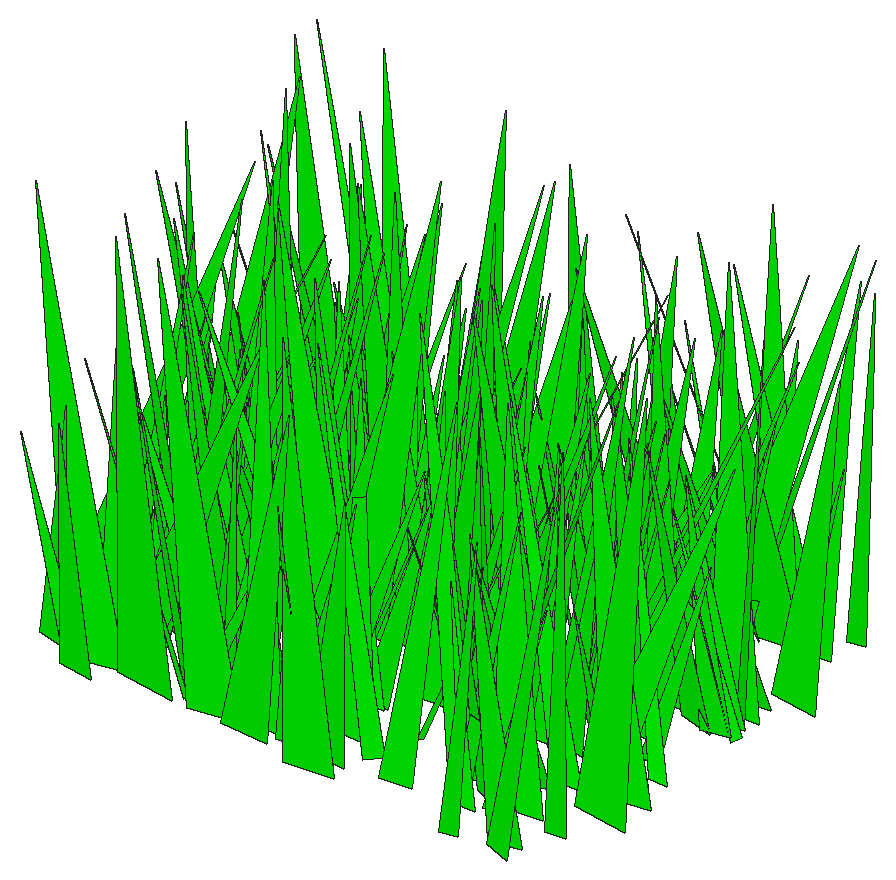
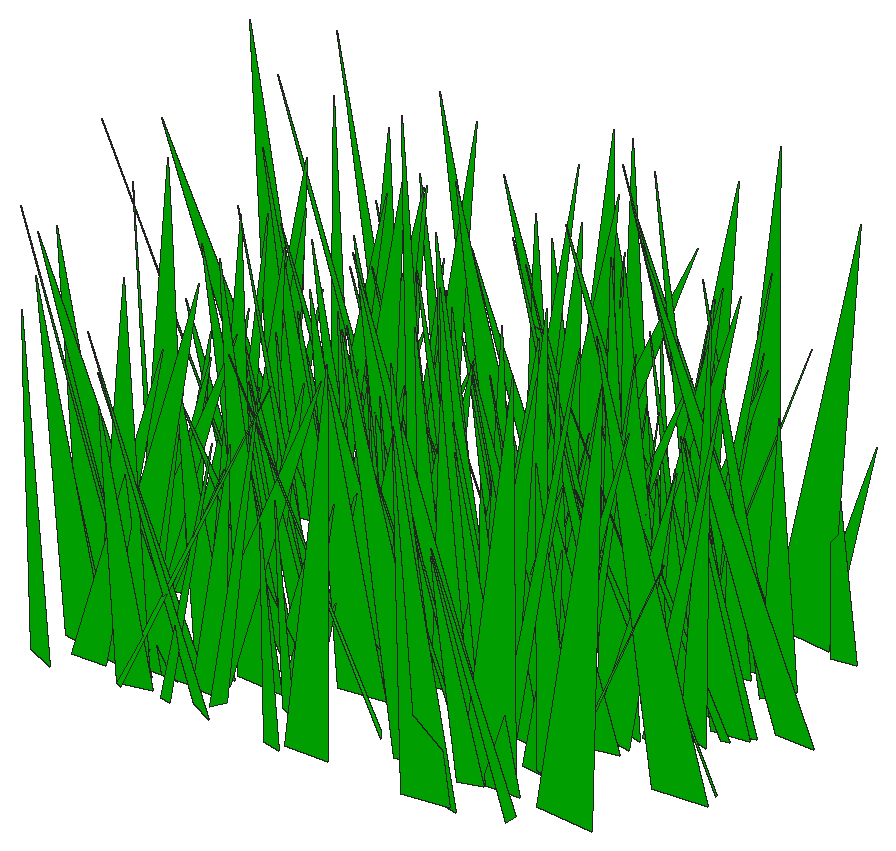
# SketchUp Ruby script. Lengths in inches.
U = 1.inch
M = Sketchup.active_model
def pt(a) = Geom::Point3d.new(a.map { |v| v * U })
def face(e, loops, mat)
  f = e.add_face(loops[0].map { |a| pt(a) })
  loops[1..].each { |l| e.add_face(l.map { |a| pt(a) }).erase! }
  f.material = f.back_material = mat if mat
  f
end
# faces: each face lists its corners as indices into pts; further lists are holes
def faces(e, pts, list, mat = nil) = list.each { |f| face(e, (f[0].is_a?(Array) ? f : [f]).map { |l| l.map { |i| pts[i] } }, mat) }
# xy, xz, yz: faces in a plane at the given z, y or x. An outline is a flat list of corners, or four numbers for a rectangle; further outlines are holes
def ring(l) = l.size == 4 ? [[l[0], l[1]], [l[2], l[1]], [l[2], l[3]], [l[0], l[3]]] : l.each_slice(2).to_a
def flat(e, list, mat, &to3) = list.each { |f| face(e, (f[0].is_a?(Array) ? f : [f]).map { |l| ring(l).map { |u, v| to3.(u, v) } }, mat) }
def xy(e, z, list, mat = nil) = flat(e, list, mat) { |x, y| [x, y, z] }
def xz(e, y, list, mat = nil) = flat(e, list, mat) { |x, z| [x, y, z] }
def yz(e, x, list, mat = nil) = flat(e, list, mat) { |y, z| [x, y, z] }
def lines(e, pts, list) = list.each { |a, b| e.add_line(pt(pts[a]), pt(pts[b])) }
# prism: a flat outline (further loops are holes) pulled along v
def prism(e, loops, v, mat = nil)
  f = face(e, loops, mat); d = Geom::Vector3d.new(v.map { |x| x * U })
  f.pushpull(f.normal.samedirection?(d) ? d.length : -d.length)
end
def box(e, o, s, mat = nil) = prism(e, [[o, [o[0] + s[0], o[1], o[2]], [o[0] + s[0], o[1] + s[1], o[2]], [o[0], o[1] + s[1], o[2]]]], [0, 0, s[2]], mat)
def at(x, y, z, deg = 0) = Geom::Transformation.translation(pt([x, y, z])) * Geom::Transformation.rotation(ORIGIN, Z_AXIS, deg.degrees)
def axes(o, x, y, z) = Geom::Transformation.new([*x, 0, *y, 0, *z, 0, *pt(o).to_a, 1])
def part(name) = M.definitions.add(name)
# library, detail: a bought-in or finely detailed component or shape, given as its bounding box
def library(name, o, s) = part(name).tap { |d| box(d.entities, o, s) }
def detail(e, o, s) = box(e.add_group.entities, o, s)
def put(e, d, t, mat = nil) = e.add_instance(d, t).tap { |i| i.material = mat if mat }
def group(e, t, mat = nil) = e.add_group.tap { |g| g.transformation = t; g.material = mat if mat }.entities
root = M.entities
M.materials.add("[0065_Lime]").color = [0, 255, 0]
c1 = part("fur_instance\#9")
p = [[0.8125,0,1.79],[0.67,-0.02,1.48],[0,-0.11,0],[0,0.11,0]]
faces(c1.entities,p,[[0,1,2,3]])
put(root,c1,axes([150.21,31.57,1.48],[1.25722,-1.1199,2.20986],[8.33837,0.21926,0.58469],[-1.17085,0.35899,6.53684]),"[0065_Lime]")
put(root,c1,axes([148.53,28.71,1.48],[1.16596,1.23629,0.95394],[-8.84406,0.14774,0.73606],[0.75159,-0.17936,7.18145]),"[0065_Lime]")
put(root,c1,axes([150.23,26.02,1.48],[6.06668,0.6304,2.794],[-4.69091,0.95672,-0.4941],[-3.14967,-0.21064,6.1175]),"[0065_Lime]")
put(root,c1,axes([151.66,29.75,1.48],[-5.19716,-0.05545,0.37346],[0.46632,-0.72225,0.69996],[0.38612,0.12586,4.18142]),"[0065_Lime]")
put(root,c1,axes([150.99,26.8,1.48],[-5.757,-0.54802,1.14363],[3.87575,-0.83147,-0.44215],[1.47149,0.04595,5.63887]),"[0065_Lime]")
put(root,c1,axes([149.74,20.19,1.48],[-1.95337,-0.61768,0.9126],[4.3473,-0.30393,-0.73637],[1.29694,0.08845,3.84276]),"[0065_Lime]")
put(root,c1,axes([150.39,22.17,1.48],[1.14069,0.81233,0.10333],[-5.7234,0.16121,-0.6625],[-0.8236,0.00482,4.74697]),"[0065_Lime]")
put(root,c1,axes([151.1,19.46,1.48],[-2.82874,0.41361,0.72305],[-3.06841,-0.39064,-0.45464],[0.1977,-0.14491,3.28939]),"[0065_Lime]")
put(root,c1,axes([149.5625,25.26,1.48],[-0.08642,0.8548,0.2891],[-6.05029,-0.01798,0.58487],[0.7252,-0.04815,4.91399]),"[0065_Lime]")
put(root,c1,axes([151.46,19.91,1.48],[-1.91109,1.18893,1.46459],[-8.63546,-0.24693,-0.73853],[-0.50999,-0.27414,7.01694]),"[0065_Lime]")
put(root,c1,axes([147.82,28.05,1.48],[6.7977,0.06806,0.24061],[-0.50567,0.95316,0.41755],[-0.2577,-0.07496,5.52761]),"[0065_Lime]")
put(root,c1,axes([149.375,25.08,1.48],[1.69963,-0.68769,1.09754],[5.06302,0.21503,-0.67286],[0.3705,0.21621,4.15998]),"[0065_Lime]")
put(root,c1,axes([148.03,24.44,1.48],[6.20339,0.92123,0.82324],[-6.63313,0.86388,0.67735],[-0.08398,-0.18379,7.3103]),"[0065_Lime]")
put(root,c1,axes([151.93,27.42,1.48],[-1.03951,-0.75241,1.22688],[5.51866,-0.11233,0.78541],[-0.70054,0.2316,4.36672]),"[0065_Lime]")
put(root,c1,axes([150.1,22.9375,1.48],[7.07255,-0.25948,1.89783],[2.19672,1.02559,-0.71773],[-2.00699,0.20815,5.90228]),"[0065_Lime]")
put(root,c1,axes([151.26,19.26,1.48],[-1.66813,-0.7076,0.17773],[4.99243,-0.2364,-0.53558],[0.69374,-0.0002,4.2816]),"[0065_Lime]")
put(root,c1,axes([152.82,29.54,1.48],[-5.91693,-0.51747,1.22347],[3.86725,-0.83703,0.51137],[0.93194,0.18795,5.64585]),"[0065_Lime]")
put(root,c1,axes([151.47,22.625,1.48],[-1.6541,0.58026,0.46138],[-4.11396,-0.24106,0.40058],[0.67048,-0.04759,3.59617]),"[0065_Lime]")
put(root,c1,axes([150.58,24.77,1.48],[0.44322,-0.57424,0.08187],[4.01648,0.05853,-0.63074],[0.76047,0.02556,3.28356]),"[0065_Lime]")
put(root,c1,axes([149.6,27.11,1.48],[3.91011,0.3967,0.2188],[-2.82089,0.53746,0.70179],[0.29127,-0.12021,3.8596]),"[0065_Lime]")
put(root,c1,axes([152.92,30.91,1.48],[-8.58835,0.29702,1.79511],[-2.03943,-1.24601,0.45255],[2.27574,0.00428,7.1801]),"[0065_Lime]")
put(root,c1,axes([149.5,25.57,1.48],[5.25428,0.28824,0.2291],[-2.06987,0.72853,0.69494],[0.05174,-0.1262,4.53512]),"[0065_Lime]")
put(root,c1,axes([152.77,27.72,1.48],[-7.60711,0.13118,1.77263],[-0.73286,-1.10889,0.66897],[2.25469,0.08217,6.19815]),"[0065_Lime]")
put(root,c1,axes([153.3,24.41,1.48],[-3.79992,-0.98927,1.54484],[7.29163,-0.51312,0.8564],[-0.05802,0.30503,6.45089]),"[0065_Lime]")
put(root,c1,axes([151.68,24.58,1.48],[-2.27555,-0.57882,0.90432],[4.13149,-0.34314,-0.48106],[1.06525,0.09437,3.79754]),"[0065_Lime]")
put(root,c1,axes([151.67,30.06,1.48],[1.69895,0.9314,0.13758],[-6.59309,0.23991,-0.55556],[-0.7036,0.00093,5.5381]),"[0065_Lime]")
put(root,c1,axes([153.14,22.14,1.48],[-7.01701,-0.40988,1.82186],[3.22627,-1.01151,0.59611],[1.76528,0.21938,6.15242]),"[0065_Lime]")
put(root,c1,axes([152.55,25.0625,1.48],[-4.44621,0.26356,0.88729],[-1.68943,-0.63982,0.76726],[1.36155,0.06678,3.84953]),"[0065_Lime]")
put(root,c1,axes([152.2,25.18,1.48],[-2.28247,0.5908,0.41408],[-4.15698,-0.32807,0.52394],[0.80995,-0.01887,3.85597]),"[0065_Lime]")
put(root,c1,axes([152.37,30.04,1.48],[1.22434,-0.58966,0.73665],[4.19745,0.19218,0.53899],[-0.90033,0.09412,3.51456]),"[0065_Lime]")
put(root,c1,axes([152.2,26.77,1.48],[5.20468,1.01749,2.17564],[-7.32825,0.79373,-0.83953],[-2.42557,-0.21476,7.20483]),"[0065_Lime]")
put(root,c1,axes([152.99,31.34,1.48],[-3.89804,1.13981,0.48533],[-8.08204,-0.55325,0.59017],[0.91298,-0.03107,7.29651]),"[0065_Lime]")
put(root,c1,axes([151.4,22.2,1.48],[2.7931,-0.51149,1.11385],[3.88515,0.37765,-0.63478],[-0.17534,0.2201,3.67771]),"[0065_Lime]")
put(root,c1,axes([151.31,32.49,1.48],[4.77893,-0.10782,0.7687],[0.96253,0.66404,-0.83809],[-0.74526,0.16622,3.8468]),"[0065_Lime]")
put(root,c1,axes([154.49,19.95,1.48],[-5.94163,-0.0114,0.58857],[0.14175,-0.83803,0.40268],[0.71419,0.07145,4.81665]),"[0065_Lime]")
put(root,c1,axes([154.0625,22.97,1.48],[-4.7246,0.83667,1.38845],[-6.15706,-0.66729,-0.38804],[0.67591,-0.23023,6.17052]),"[0065_Lime]")
put(root,c1,axes([151.69,28.04,1.48],[1.37139,0.69688,1.32194],[-5.18801,0.1564,0.79821],[0.56668,-0.25461,4.10859]),"[0065_Lime]")
put(root,c1,axes([153.34,25.2,1.48],[-5.29419,-0.13055,1.3807],[0.69726,-0.77682,-0.69241],[1.80506,-0.08284,4.317]),"[0065_Lime]")
put(root,c1,axes([153.37,22.8125,1.48],[2.15496,-0.91793,1.49343],[6.61566,0.34441,0.77743],[-1.50903,0.19908,5.54098]),"[0065_Lime]")
put(root,c1,axes([153.98,20.64,1.48],[-5.1385,-0.24778,1.28974],[2.01253,-0.73689,0.56143],[1.25422,0.16729,4.38316]),"[0065_Lime]")
put(root,c1,axes([153.22,19.78,1.48],[-2.90433,-1.24946,0.66929],[8.85228,-0.41883,-0.78424],[1.17414,0.06709,7.56824]),"[0065_Lime]")
put(root,c1,axes([154.28,29.67,1.48],[-4.98617,0.96466,0.22805],[-6.80156,-0.6999,0.81315],[0.9729,0.05094,6.85354]),"[0065_Lime]")
put(root,c1,axes([152.45,31.41,1.48],[2.76752,0.7426,1.5538],[-5.60494,0.38625,0.41954],[-0.40309,-0.2722,4.8343]),"[0065_Lime]")
put(root,c1,axes([153.29,24.38,1.48],[3.23255,1.12177,0.91797],[-7.93125,0.47314,-0.89514],[-1.44883,-0.08725,6.9483]),"[0065_Lime]")
put(root,c1,axes([155.05,20.88,1.48],[-4.22603,0.49222,0.84553],[-3.65264,-0.57489,-0.8648],[0.09461,-0.20851,4.38031]),"[0065_Lime]")
put(root,c1,axes([152.54,22.4375,1.48],[-6.65901,-0.60054,3.4818],[4.41883,-1.09385,-0.73045],[4.13056,0.20204,6.39454]),"[0065_Lime]")
put(root,c1,axes([154.57,21.95,1.48],[-4.95723,-0.58308,1.86579],[4.58455,-0.7084,0.64091],[1.20914,0.29543,5.2193]),"[0065_Lime]")
put(root,c1,axes([153.91,28.92,1.48],[1.19026,-1.17819,0.89337],[8.42049,0.17946,0.50789],[-0.77731,0.13995,6.86982]),"[0065_Lime]")
put(root,c1,axes([155,28.43,1.48],[-2.70053,0.65221,0.5112],[-4.68129,-0.37245,-0.43922],[-0.15546,-0.11436,4.34586]),"[0065_Lime]")
put(root,c1,axes([154.74,22.28,1.48],[-0.09931,0.5604,1.34787],[-4.22968,0.03441,-0.68558],[-0.87206,-0.23071,3.17172]),"[0065_Lime]")
put(root,c1,axes([153.39,31.62,1.48],[-0.93809,0.58408,0.77313],[-4.13394,-0.15809,0.68343],[1.04486,-0.10109,3.39807]),"[0065_Lime]")
put(root,c1,axes([153.47,32.93,1.48],[3.88665,0.88606,0.82098],[-6.27534,0.5607,-0.62157],[-1.18328,-0.06323,5.99301]),"[0065_Lime]")
put(root,c1,axes([153.16,28.52,1.48],[6.1171,0.38451,1.31943],[-2.62844,0.88923,-0.62084],[-1.79173,0.00826,5.41541]),"[0065_Lime]")
put(root,c1,axes([152.56,28.87,1.48],[5.63977,-0.53349,1.08494],[3.93723,0.79823,-0.38896],[-0.8316,0.16121,5.51639]),"[0065_Lime]")
put(root,c1,axes([152.04,23.66,1.48],[7.52504,-0.40401,1.05935],[3.01872,1.05939,-0.64933],[-0.92197,0.17114,6.52028]),"[0065_Lime]")
put(root,c1,axes([155.03,28.26,1.48],[0.59201,0.58476,1.08118],[-4.25043,0.12065,-0.64666],[-1.00931,-0.16507,3.3574]),"[0065_Lime]")
put(root,c1,axes([155.01,28.47,1.48],[0.96048,-1.01899,1.69173],[7.46402,0.17116,0.6507],[-1.09591,0.27264,5.91445]),"[0065_Lime]")
put(root,c1,axes([152,21.01,1.48],[4.29987,-0.9551,0.05596],[6.75404,0.59903,-0.77291],[0.76652,0.0795,6.49641]),"[0065_Lime]")
put(root,c1,axes([152.62,20.95,1.48],[8.0927,0.46333,1.06589],[-3.15987,1.14971,-0.87297],[-1.61382,0.07227,7.05431]),"[0065_Lime]")
put(root,c1,axes([153.75,33.09,1.48],[-1.62171,-1.07188,1.79012],[7.78346,-0.27686,-0.88962],[1.56469,0.26629,6.28074]),"[0065_Lime]")
put(root,c1,axes([154.79,26.18,1.48],[-4.36605,0.61742,1.11153],[-4.25765,-0.64245,0.8928],[1.74524,-0.02273,4.95874]),"[0065_Lime]")
put(root,c1,axes([155.65,19.68,1.48],[-1.94782,1.08033,2.13894],[-8.12134,-0.24672,-0.71766],[-0.25925,-0.38804,6.41123]),"[0065_Lime]")
put(root,c1,axes([153.1,25.34,1.48],[7.27364,0.40153,1.17201],[-2.80324,1.04193,-0.45087],[-1.54379,-0.00013,6.34066]),"[0065_Lime]")
put(root,c1,axes([156.43,22.8,1.48],[-3.8382,-0.58681,0.45736],[4.21143,-0.53066,0.56905],[-0.14002,0.12458,4.57844]),"[0065_Lime]")
put(root,c1,axes([154.47,21.11,1.48],[4.87225,0.34571,1.1291],[-2.24817,0.71001,-0.86587],[-1.71039,0.05154,4.3545]),"[0065_Lime]")
put(root,c1,axes([153.71,28.13,1.48],[6.11243,-0.17924,1.00481],[1.18473,0.87514,0.46261],[-1.32265,-0.04443,5.05792]),"[0065_Lime]")
put(root,c1,axes([155.28,28.05,1.48],[3.31211,0.88961,2.03434],[-6.59862,0.51558,-0.44678],[-1.67156,-0.27257,5.79464]),"[0065_Lime]")
put(root,c1,axes([155.69,22.54,1.48],[-4.01851,-0.26178,0.86011],[1.64378,-0.57937,-0.82742],[1.37355,-0.0725,3.50657]),"[0065_Lime]")
put(root,c1,axes([154.59,22.0625,1.48],[0.72977,0.78162,0.57749],[-5.58535,0.09237,0.48082],[0.49893,-0.10926,4.53795]),"[0065_Lime]")
put(root,c1,axes([155.41,20.64,1.48],[4.36716,0.41112,1.43193],[-2.78469,0.66124,-0.74241],[-1.97604,-0.02322,4.21088]),"[0065_Lime]")
put(root,c1,axes([155.51,27.97,1.48],[-1.45328,0.63254,0.23399],[-4.4581,-0.20789,0.51111],[0.68666,-0.01095,3.81356]),"[0065_Lime]")
put(root,c1,axes([156.1,26.46,1.48],[2.62887,-0.64008,1.36069],[4.52414,0.41997,0.83669],[-1.75489,0.12384,4.19535]),"[0065_Lime]")
put(root,c1,axes([153.91,24.93,1.48],[7.1511,0.42243,1.44974],[-3.22222,1.01779,0.57861],[-1.35324,-0.19119,6.2833]),"[0065_Lime]")
put(root,c1,axes([156.25,24.38,1.48],[-4.5477,-0.44224,0.78798],[3.00612,-0.6523,-0.78821],[1.34408,-0.03741,4.42899]),"[0065_Lime]")
put(root,c1,axes([156.93,24.41,1.48],[-4.25137,-0.11381,0.7346],[0.70114,-0.60795,-0.47137],[0.98995,-0.05818,3.48862]),"[0065_Lime]")
put(root,c1,axes([157.52,22.875,1.48],[-3.05967,1.15342,1.43101],[-8.39453,-0.41829,-0.57803],[-0.06673,-0.26645,7.10209]),"[0065_Lime]")
put(root,c1,axes([154.54,20.49,1.48],[4.34245,-0.25449,0.24626],[1.83456,0.60595,-0.42071],[-0.07822,0.08349,3.80391]),"[0065_Lime]")
put(root,c1,axes([155.68,27.54,1.48],[4.35013,-0.28743,1.42244],[2.42467,0.62126,-0.69959],[-1.16754,0.21925,3.84702]),"[0065_Lime]")
put(root,c1,axes([159.02,21.07,1.48],[-6.38904,0.61876,0.57947],[-4.46057,-0.88741,-0.78763],[0.03017,-0.16887,6.26235]),"[0065_Lime]")
put(root,c1,axes([154.86,30.11,1.48],[4.74666,-0.04762,0.25778],[0.273,0.65675,0.73971],[-0.37519,-0.12463,3.79949]),"[0065_Lime]")
put(root,c1,axes([157.08,27.11,1.48],[2.84865,-0.52026,1.67989],[3.77077,0.47073,0.65443],[-1.93773,0.15119,3.74309]),"[0065_Lime]")
put(root,c1,axes([155.17,31.63,1.48],[3.44929,-0.96318,1.24677],[7.02359,0.47122,-0.65808],[0.05182,0.24343,6.20689]),"[0065_Lime]")
put(root,c1,axes([157.04,23.68,1.48],[2.21239,-1.09524,0.71005],[7.7374,0.32563,0.87993],[-1.28291,0.0752,6.53144]),"[0065_Lime]")
put(root,c1,axes([155.66,25.78,1.48],[1.86242,1.23841,1.6702],[-9.03066,0.23548,0.812],[0.57982,-0.3103,7.28197]),"[0065_Lime]")
put(root,c1,axes([156.99,27.99,1.48],[-2.51417,0.7595,0.82808],[-5.38849,-0.37166,0.59783],[1.10214,-0.08453,4.81187]),"[0065_Lime]")
put(root,c1,axes([155.85,28.87,1.48],[4.03392,0.13604,0.65811],[-1.12303,0.56073,0.67048],[-0.57506,-0.14075,3.30713]),"[0065_Lime]")
put(root,c1,axes([157.08,19.9375,1.48],[-5.74935,0.79673,2.24985],[-5.78488,-0.8756,0.60916],[2.51672,-0.19253,6.53989]),"[0065_Lime]")
put(root,c1,axes([156.45,20.41,1.48],[1.33827,0.56664,0.79232],[-4.14478,0.17655,0.40096],[0.17525,-0.15141,3.43266]),"[0065_Lime]")
put(root,c1,axes([155.71,28.67,1.48],[6.76364,0.79155,0.61763],[-5.57345,0.95612,-0.67742],[-1.11578,0.02228,7.1277]),"[0065_Lime]")
put(root,c1,axes([157.82,33.09,1.48],[-2.77103,-0.97335,1.25567],[7.01497,-0.41094,-0.43147],[1.07485,0.17262,6.0532]),"[0065_Lime]")
put(root,c1,axes([157.4375,26.92,1.48],[-3.77794,-0.77552,2.00029],[5.60458,-0.60205,-0.81789],[2.25733,0.19687,5.37846]),"[0065_Lime]")
put(root,c1,axes([156.89,19.44,1.48],[1.37878,-0.99747,0.34502],[7.09084,0.18825,-0.51148],[0.53777,0.07516,5.85967]),"[0065_Lime]")
put(root,c1,axes([156.82,24.74,1.48],[4.14105,0.17888,0.24105],[-1.19709,0.5746,-0.68179],[-0.52478,0.10084,3.45737]),"[0065_Lime]")
put(root,c1,axes([157.43,27.69,1.48],[-0.93215,-0.68203,0.71127],[4.80565,-0.15372,-0.77211],[1.10852,0.09287,3.94537]),"[0065_Lime]")
put(root,c1,axes([158.05,19.77,1.48],[2.48914,0.47221,0.78327],[-3.31561,0.37154,-0.53433],[-1.10772,-0.051,3.35944]),"[0065_Lime]")
put(root,c1,axes([158,32.54,1.48],[3.85428,-0.39067,1.02302],[2.60057,0.56949,0.80481],[-1.59642,-0.01552,3.78095]),"[0065_Lime]")
put(root,c1,axes([157.66,27.73,1.48],[-3.33198,-0.73114,1.78516],[5.26432,-0.53174,-0.79654],[2.0437,0.17767,4.96225]),"[0065_Lime]")
put(root,c1,axes([157.09,26.79,1.48],[6.59633,-0.37232,1.32896],[2.57865,0.9549,0.4961],[-1.74374,0.00366,5.76091]),"[0065_Lime]")
put(root,c1,axes([159.07,29.14,1.48],[-1.36662,0.81262,1.41498],[-6.03317,-0.17268,-0.53223],[-0.26587,-0.25847,4.80419]),"[0065_Lime]")
put(root,c1,axes([158.8,22.74,1.48],[-3.81542,0.26019,0.86224],[-1.75669,-0.55629,0.48182],[1.21089,0.01279,3.41586]),"[0065_Lime]")
put(root,c1,axes([157.75,21.02,1.48],[0.08378,-0.62265,1.23264],[4.58031,-0.03347,-0.77253],[0.97556,0.21062,3.5212]),"[0065_Lime]")
put(root,c1,axes([159.17,19.1875,1.48],[-5.01131,-0.31768,1.31516],[2.15751,-0.73992,-0.54964],[1.75227,0.0025,4.43797]),"[0065_Lime]")
put(root,c1,axes([158.03,25.77,1.48],[0.62182,-1.01356,2.03113],[7.61741,0.0599,-0.54129],[0.48777,0.3566,5.864]),"[0065_Lime]")
put(root,c1,axes([157.75,29.07,1.48],[0.73601,0.92968,0.15776],[-6.56443,0.09901,0.71102],[0.84787,-0.04044,5.36795]),"[0065_Lime]")
put(root,c1,axes([157.75,29.07,1.48],[6.16283,-0.34825,1.09341],[2.3371,0.88497,0.72934],[-1.57707,-0.04944,5.35364]),"[0065_Lime]")
put(root,c1,axes([157.12,21.43,1.48],[5.37063,-0.71436,0.98527],[5.2031,0.75374,-0.45291],[-0.48931,0.17425,5.99823]),"[0065_Lime]")
put(root,c1,axes([159.49,18.94,1.48],[0.90646,1.05728,2.23153],[-7.94694,0.16683,-0.51282],[-0.99268,-0.37014,6.14313]),"[0065_Lime]")
put(root,c1,axes([159.85,31.13,1.48],[-2.02214,-0.4602,1.55049],[3.78872,-0.25099,0.77303],[0.06806,0.29914,3.03388]),"[0065_Lime]")
put(root,c1,axes([158.8125,33.35,1.48],[3.63938,-0.28882,0.70916],[1.836,0.52046,0.86867],[-1.2704,-0.07523,3.28697]),"[0065_Lime]")
put(root,c1,axes([159.07,28.38,1.48],[5.33549,-0.00441,1.71323],[-0.19852,0.80132,0.47811],[-2.09708,-0.08707,4.31362]),"[0065_Lime]")
put(root,c1,axes([159.45,21.03,1.48],[-3.7831,0.77084,1.5157],[-5.55173,-0.57174,0.57511],[1.65628,-0.15577,5.38973]),"[0065_Lime]")
put(root,c1,axes([156.92,31.03,1.48],[6.76729,0.10195,0.1585],[-0.70576,0.94782,-0.49125],[-0.25738,0.08151,5.5143]),"[0065_Lime]")
put(root,c1,axes([158.68,29.63,1.48],[0.17582,1.00315,1.97279],[-7.49282,-0.01471,0.69248],[0.83952,-0.34138,5.76727]),"[0065_Lime]")
put(root,c1,axes([160.22,29.76,1.48],[-3.48515,-0.3614,0.52969],[2.52534,-0.4982,-0.39634],[0.81321,-0.00172,3.50084]),"[0065_Lime]")
put(root,c1,axes([160.48,20.52,1.48],[-6.88774,0.31659,2.09147],[-2.67648,-1.00497,-0.73443],[2.12691,-0.2394,5.84877]),"[0065_Lime]")
put(root,c1,axes([158.57,22.91,1.48],[2.40701,-0.54403,0.87273],[4.01575,0.32054,-0.63249],[0.12021,0.18543,3.6539]),"[0065_Lime]")
put(root,c1,axes([159.36,27.35,1.48],[4.32162,0.14707,1.47428],[-1.36574,0.64092,0.50649],[-1.58591,-0.15119,3.58124]),"[0065_Lime]")
put(root,c1,axes([159.58,31.67,1.48],[3.34459,0.33392,0.8981],[-2.22283,0.49477,-0.68723],[-1.38753,0.01229,3.2658]),"[0065_Lime]")
put(root,c1,axes([159.68,23.9,1.48],[2.13037,0.80826,0.47754],[-5.70408,0.30817,-0.6417],[-0.94538,-0.03804,4.94791]),"[0065_Lime]")
put(root,c1,axes([158.33,21.3125,1.48],[4.876,-0.4389,0.67642],[3.21419,0.68071,-0.52969],[-0.34094,0.14047,4.68027]),"[0065_Lime]")
put(root,c1,axes([159.48,19.66,1.48],[-0.02954,-0.83486,0.00385],[5.90029,-0.0042,-0.56694],[0.697,0.00017,4.79943]),"[0065_Lime]")
put(root,c1,axes([160.875,23.75,1.48],[-0.21953,-0.61828,1.00526],[4.53877,-0.00911,0.46815],[-0.53595,0.17614,3.55279]),"[0065_Lime]")
put(root,c1,axes([161.34,32.46,1.48],[-6.18917,0.29467,1.32721],[-1.89256,-0.89684,0.83288],[1.86495,0.06779,5.24982]),"[0065_Lime]")
put(root,c1,axes([160.19,25.93,1.48],[-2.07009,0.78451,1.16812],[-5.58694,-0.32586,0.7825],[1.42055,-0.13838,4.77975]),"[0065_Lime]")
put(root,c1,axes([159.73,28.08,1.48],[2.82583,0.66361,1.00797],[-4.87824,0.39214,0.39764],[-0.20377,-0.18499,4.45892]),"[0065_Lime]")
put(root,c1,axes([160.02,25.77,1.48],[3.713,0.99794,0.24666],[-7.04712,0.52307,-0.72572],[-0.93084,0.0206,6.4781]),"[0065_Lime]")
put(root,c1,axes([162.45,31.36,1.48],[-3.22237,-0.82877,0.32491],[5.89725,-0.44624,0.55558],[-0.40993,0.0951,5.43851]),"[0065_Lime]")
put(root,c1,axes([160.74,24.46,1.48],[7.27768,0.70266,2.45612],[-4.97893,1.10065,-0.79013],[-3.05494,-0.11993,7.13887]),"[0065_Lime]")
put(root,c1,axes([161.88,28.5,1.48],[1.27687,-0.53222,0.84645],[3.71143,0.21382,0.80059],[-1.28595,0.08864,3.15109]),"[0065_Lime]")
put(root,c1,axes([161.99,22.64,1.48],[1.62431,0.52295,1.23034],[-3.78814,0.2757,-0.61783],[-1.33724,-0.1458,3.24467]),"[0065_Lime]")
put(root,c1,axes([164.1,33.27,1.48],[-7.10131,-0.20486,0.27162],[1.4263,-0.9961,-0.50184],[0.45012,-0.07561,5.87538]),"[0065_Lime]")
put(root,c1,axes([161.93,32.16,1.48],[1.30412,-0.636,1.13663],[4.65028,0.21067,0.41991],[-0.90197,0.16659,3.80833]),"[0065_Lime]")
put(root,c1,axes([160.4,23.77,1.48],[4.733,0.43098,1.08504],[-3.27693,0.66255,0.63916],[-0.66941,-0.19616,4.54281]),"[0065_Lime]")
put(root,c1,axes([162.48,24.92,1.48],[2.45379,-1.05185,2.01507],[7.68053,0.40131,0.83128],[-1.78315,0.2811,6.35347]),"[0065_Lime]")
put(root,c1,axes([162.6,33.14,1.48],[4.3999,-0.17063,2.14228],[0.8485,0.71877,0.7653],[-2.77324,-0.0508,3.633]),"[0065_Lime]")
put(root,c1,axes([162.84,24.55,1.48],[-0.10683,-1.0819,1.49345],[7.85264,0.0179,0.80624],[-0.99361,0.25781,6.21126]),"[0065_Lime]")
put(root,c1,axes([159.77,26.73,1.48],[7.07472,-0.30503,0.45384],[2.09949,0.99278,0.70477],[-0.7846,-0.09388,5.97807]),"[0065_Lime]")
put(root,c1,axes([163.05,21.28,1.48],[-6.45058,0.75101,1.40498],[-5.31919,-0.93551,0.59816],[1.80395,-0.07301,6.78768]),"[0065_Lime]")
put(root,c1,axes([161.14,30.95,1.48],[4.93648,-0.90033,0.47068],[6.33044,0.69806,0.81465],[-1.14583,-0.0222,6.52854]),"[0065_Lime]")
put(root,c1,axes([160.76,22.16,1.48],[4.86095,0.21201,0.17688],[-1.44213,0.67267,-0.79553],[-0.49399,0.12248,4.0629]),"[0065_Lime]")
put(root,c1,axes([163.87,21.4,1.48],[-4.27441,-0.20957,0.43597],[1.56409,-0.59276,0.59836],[0.25529,0.12276,3.63349]),"[0065_Lime]")
put(root,c1,axes([162.34,25.53,1.48],[4.70108,-0.25479,1.3267],[1.66934,0.699,0.58449],[-1.77799,-0.01739,4.0566]),"[0065_Lime]")
put(root,c1,axes([161.8,28.1875,1.48],[3.94403,-0.29272,1.22665],[2.44737,0.54639,-0.83732],[-0.78996,0.23131,3.53018]),"[0065_Lime]")
put(root,c1,axes([161.76,19.84,1.48],[6.27653,-0.56131,1.9733],[4.35736,0.90921,-0.50377],[-1.68976,0.25962,6.03067]),"[0065_Lime]")
put(root,c1,axes([163.73,25.69,1.48],[-4.32716,-0.14207,0.93109],[1.20494,-0.61452,0.56318],[0.93837,0.13398,3.57042]),"[0065_Lime]")
put(root,c1,axes([162.3,21.78,1.48],[3.99426,-0.08054,0.89401],[0.33962,0.57224,0.72347],[-1.19212,-0.10682,3.20153]),"[0065_Lime]")
put(root,c1,axes([163.44,28.15,1.48],[-0.08905,-0.71246,0.02734],[5.03606,-0.01188,0.47934],[-0.58863,0.00615,4.09688]),"[0065_Lime]")
put(root,c1,axes([162.97,22.4,1.48],[-5.24465,-0.38203,1.74047],[2.60138,-0.79542,-0.66397],[2.28097,0.02874,4.75911]),"[0065_Lime]")
put(root,c1,axes([162.41,31.25,1.48],[-0.48008,0.82158,1.03279],[-5.92595,-0.08997,0.57563],[0.82477,-0.16819,4.73702]),"[0065_Lime]")
put(root,c1,axes([164.3,32.1,1.48],[-4.3871,-0.19517,0.24351],[1.30615,-0.60772,-0.75198],[0.5592,-0.11167,3.66678]),"[0065_Lime]")
put(root,c1,axes([162.84,27.07,1.48],[3.52197,0.53755,1.0826],[-3.8503,0.52126,-0.38527],[-1.25741,-0.09048,4.21207]),"[0065_Lime]")
put(root,c1,axes([161.47,33.04,1.48],[6.36325,0.44515,0.48875],[-3.08037,0.89445,-0.7635],[-0.95299,0.08119,5.73129]),"[0065_Lime]")
put(root,c1,axes([161.53,29.14,1.48],[2.90675,0.50344,0.00324],[-3.52548,0.40179,0.67076],[0.63791,-0.07343,3.69231]),"[0065_Lime]")
put(root,c1,axes([162.43,27.37,1.48],[4.14585,0.52928,0.45365],[-3.71118,0.58759,-0.53203],[-0.85196,0.01602,4.52508]),"[0065_Lime]")
put(root,c1,axes([162.32,27.16,1.48],[6.94652,0.37767,1.39934],[-2.60208,1.00559,-0.54778],[-1.84726,0.00371,6.03376]),"[0065_Lime]")
put(root,c1,axes([164.08,20.74,1.48],[-4.04362,-0.39291,0.81055],[2.61577,-0.5835,-0.84398],[1.40328,-0.04451,3.90885]),"[0065_Lime]")
put(root,c1,axes([164.94,22.07,1.48],[-2.53062,-0.46533,0.96511],[3.51175,-0.32226,0.88587],[-0.20433,0.22448,3.27234]),"[0065_Lime]")
put(root,c1,axes([164.14,19.95,1.48],[-3.57367,0.28451,0.82857],[-1.93357,-0.52213,0.4898],[1.18252,0.00605,3.30489]),"[0065_Lime]")
put(root,c1,axes([162.79,27.81,1.48],[4.89673,0.21076,1.26247],[-1.84085,0.69011,0.8637],[-1.12682,-0.21155,4.07519]),"[0065_Lime]")
put(root,c1,axes([162.75,28.01,1.48],[4.41188,-0.1975,0.4553],[1.28236,0.61686,0.74461],[-0.8027,-0.10005,3.69205]),"[0065_Lime]")
put(root,c1,axes([165.06,32.17,1.48],[-1.98925,-1.06537,0.82494],[7.63847,-0.26885,0.5525],[-0.40606,0.16175,6.35183]),"[0065_Lime]")
put(root,c1,axes([162.36,31.875,1.48],[5.16536,0.42475,0.11361],[-2.96716,0.71858,-0.76411],[-0.59364,0.10417,4.80778]),"[0065_Lime]")
put(root,c1,axes([163.36,24.0625,1.48],[5.01452,-0.34583,1.70346],[2.85906,0.72798,-0.61626],[-1.50613,0.23052,4.50167]),"[0065_Lime]")
put(root,c1,axes([163.02,28.34,1.48],[3.76193,0.77499,1.68395],[-5.86723,0.52388,0.59332],[-0.52868,-0.29935,5.39791]),"[0065_Lime]")
put(root,c1,axes([163.69,33.08,1.48],[-1.05758,0.77565,0.51155],[-5.47512,-0.16078,0.6795],[0.94259,-0.0636,4.52089]),"[0065_Lime]")
put(root,c1,axes([165.58,32.72,1.48],[-4.80035,0.64391,1.12396],[-4.74034,-0.67761,-0.3872],[0.66117,-0.18315,5.38424]),"[0065_Lime]")
put(root,c1,axes([165.42,22.59,1.48],[-5.88284,0.57056,0.79662],[-3.95604,-0.83738,0.76785],[1.34018,0.0327,5.76342]),"[0065_Lime]")
put(root,c1,axes([163.26,32.13,1.48],[4.11136,-0.30146,0.41458],[2.0652,0.57953,0.57016],[-0.77289,-0.0551,3.72882]),"[0065_Lime]")
put(root,c1,axes([164.62,32.43,1.48],[0.91477,1.18598,0.33295],[-8.41057,0.13337,-0.63027],[-0.81515,-0.0452,6.87664]),"[0065_Lime]")
put(root,c1,axes([163.1875,25.34,1.48],[5.89541,0.66728,1.89542],[-5.09936,0.84727,0.49912],[-1.406,-0.27498,6.13735]),"[0065_Lime]")
put(root,c1,axes([163.48,20.47,1.48],[4.83151,0.46661,0.72861],[-3.20966,0.68969,-0.71819],[-1.2357,0.03295,4.71432]),"[0065_Lime]")
put(root,c1,axes([164.63,27.74,1.48],[2.57063,0.96147,1.87784],[-7.07055,0.40511,-0.54642],[-1.46795,-0.26757,5.92033]),"[0065_Lime]")
put(root,c1,axes([164.19,24.18,1.48],[-0.58799,-0.58466,1.09248],[4.2726,-0.11724,-0.58092],[0.92759,0.16941,3.36829]),"[0065_Lime]")
put(root,c1,axes([165.28,20.65,1.48],[0.01961,1.11675,0.33408],[-7.93867,0.00676,-0.44943],[-0.55427,-0.05738,6.44889]),"[0065_Lime]")
put(root,c1,axes([165.36,25.92,1.48],[1.84696,0.76569,2.19674],[-5.90868,0.31983,-0.44867],[-1.44002,-0.33026,4.65849]),"[0065_Lime]")
put(root,c1,axes([164.6,18.54,1.48],[4.33727,0.51939,1.01468],[-3.5568,0.63417,-0.81825],[-1.60246,-0.00178,4.56256]),"[0065_Lime]")
put(root,c1,axes([166.59,29.17,1.48],[-2.77663,-0.74073,0.29677],[5.27266,-0.3846,0.47298],[-0.34622,0.08329,4.82315]),"[0065_Lime]")
put(root,c1,axes([162.83,22.5,1.48],[8.23535,-0.10277,0.86549],[0.61856,1.16135,0.72687],[-1.13335,-0.11296,6.68571]),"[0065_Lime]")
put(root,c1,axes([163.23,32.11,1.48],[3.76121,1.09354,0.10024],[-7.76708,0.52612,0.50025],[0.50029,-0.05316,7.01288]),"[0065_Lime]")
put(root,c1,axes([164.58,20.29,1.48],[3.67408,0.33491,0.29663],[-2.30063,0.51489,-0.62624],[-0.72162,0.06362,3.50682]),"[0065_Lime]")
put(root,c1,axes([166.15,19.01,1.48],[1.00885,0.75296,1.36212],[-5.47515,0.18481,-0.74017],[-1.24095,-0.20325,4.37302]),"[0065_Lime]")
put(root,c1,axes([166.03,27.34,1.48],[-3.28427,-0.675,0.00443],[4.72019,-0.45365,-0.87555],[0.89159,-0.08475,4.65163]),"[0065_Lime]")
put(root,c1,axes([166.08,29.38,1.48],[3.46935,-0.23904,1.63354],[1.57387,0.56266,0.54738],[-2.10949,0.02665,3.09497]),"[0065_Lime]")
put(root,c1,axes([163.74,32.41,1.48],[8.11011,0.2031,1.09099],[-1.5884,1.14562,0.66586],[-1.16839,-0.14764,6.66766]),"[0065_Lime]")
put(root,c1,axes([166.53,23.8125,1.48],[0.93843,-0.82992,1.49377],[6.10157,0.16696,0.57221],[-1.01295,0.23686,4.83065]),"[0065_Lime]")
put(root,c1,axes([162.91,27.62,1.48],[8.60852,0.24839,0.43342],[-1.79881,1.20883,0.42507],[-0.41572,-0.0871,7.13573]),"[0065_Lime]")
put(root,c1,axes([166.97,27.77,1.48],[-3.24819,0.41663,1.03342],[-3.17568,-0.45748,-0.42401],[0.56592,-0.17582,3.55213]),"[0065_Lime]")
put(root,c1,axes([166.48,28.41,1.48],[3.88111,-0.84604,3.84178],[7.37983,0.61064,-0.42666],[-2.02398,0.60416,5.81116]),"[0065_Lime]")
put(root,c1,axes([166.75,27.28,1.48],[0.33656,-0.6227,1.35623],[4.68815,0.0767,0.41028],[-0.66263,0.22638,3.59163]),"[0065_Lime]")
put(root,c1,axes([167.25,22.85,1.48],[-1.17104,1.06089,0.41762],[-7.55222,-0.15924,-0.45654],[-0.4774,-0.08322,6.19779]),"[0065_Lime]")
put(root,c1,axes([167.41,27.36,1.48],[-4.00955,0.13486,0.80546],[-1.19075,-0.55437,-0.81172],[0.69548,-0.17168,3.25383]),"[0065_Lime]")
put(root,c1,axes([166.03,32.22,1.48],[3.31058,0.99946,0.10438],[-7.05278,0.46373,-0.78618],[-0.93011,0.04109,6.33294]),"[0065_Lime]")
put(root,c1,axes([167.21,24.24,1.48],[-5.70838,0.31833,1.36654],[-2.09136,-0.83532,0.74022],[1.89232,0.0371,4.94041]),"[0065_Lime]")
put(root,c1,axes([166.66,33.43,1.48],[5.40894,0.52078,1.6119],[-3.53918,0.80919,-0.90266],[-2.26641,-0.02074,5.25648]),"[0065_Lime]")
put(root,c1,axes([166.87,20.29,1.48],[5.63384,0.57169,1.91878],[-3.93812,0.85623,-0.89795],[-2.57063,-0.05879,5.58086]),"[0065_Lime]")
put(root,c1,axes([167.47,22.09,1.48],[-2.42091,-0.49345,0.04458],[3.47178,-0.33765,-0.49385],[0.53069,-0.04215,3.43411]),"[0065_Lime]")
put(root,c1,axes([166.23,31.33,1.48],[4.1663,-0.23199,0.55269],[1.57542,0.59177,0.46591],[-0.83992,-0.0408,3.61541]),"[0065_Lime]")
put(root,c1,axes([166.22,18.58,1.48],[6.37688,0.49097,1.88787],[-3.84799,0.92094,0.57436],[-1.66964,-0.24731,5.88666]),"[0065_Lime]")
put(root,c1,axes([167.05,27.96,1.48],[-6.47578,-0.19807,2.92186],[2.02611,-1.01373,0.66844],[3.28404,0.23486,5.34922]),"[0065_Lime]")
put(root,c1,axes([166.3125,25.01,1.48],[3.43714,-0.34607,0.72259],[2.59105,0.47919,-0.46437],[-0.37572,0.13867,3.40795]),"[0065_Lime]")
put(root,c1,axes([167.27,21.71,1.48],[-2.04396,-1.06517,2.71863],[8.07075,-0.36518,-0.77961],[1.86938,0.41195,6.33837]),"[0065_Lime]")
put(root,c1,axes([166.05,23.125,1.48],[3.6803,0.90591,0.32841],[-6.41848,0.5055,0.86557],[0.72741,-0.123,5.97597]),"[0065_Lime]")
put(root,c1,axes([167.4,29.8,1.48],[-0.08945,-0.9093,1.65021],[6.70239,-0.0553,-0.78071],[1.03349,0.27994,5.20592]),"[0065_Lime]")
